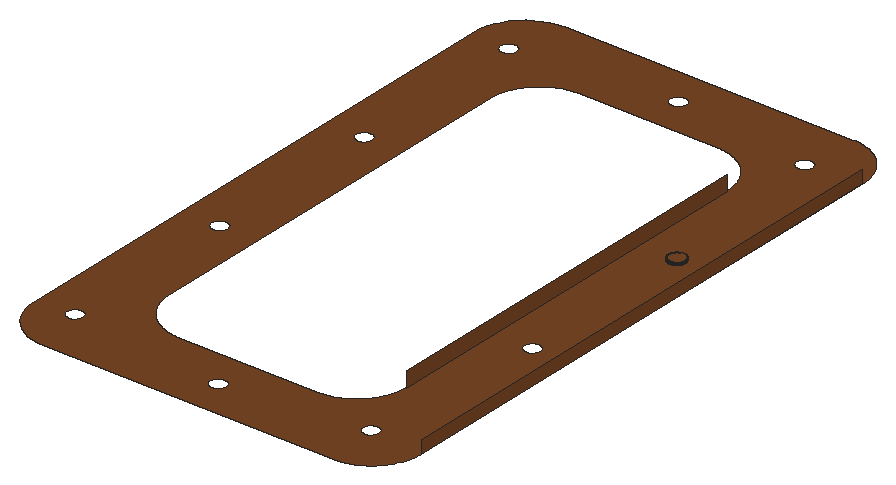
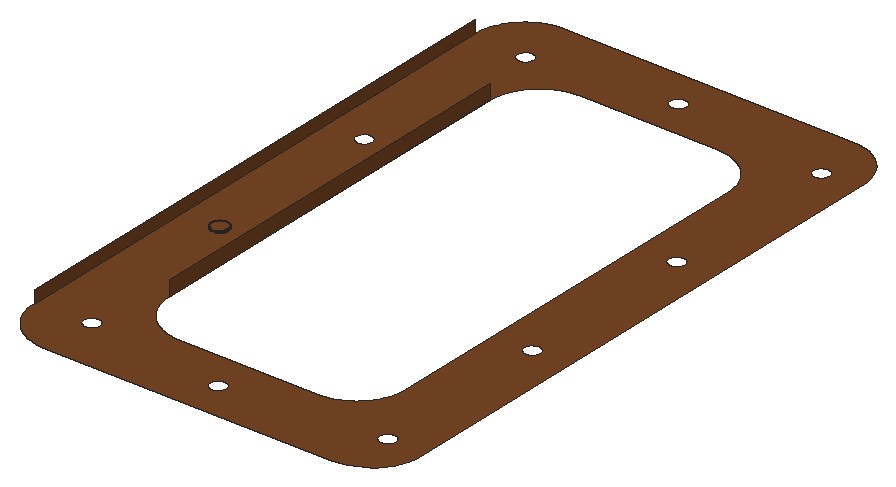
# SketchUp Ruby script. Lengths in inches.
U = 1.inch
M = Sketchup.active_model
def pt(a) = Geom::Point3d.new(a.map { |v| v * U })
def face(e, loops, mat)
  f = e.add_face(loops[0].map { |a| pt(a) })
  loops[1..].each { |l| e.add_face(l.map { |a| pt(a) }).erase! }
  f.material = f.back_material = mat if mat
  f
end
# faces: each face lists its corners as indices into pts; further lists are holes
def faces(e, pts, list, mat = nil) = list.each { |f| face(e, (f[0].is_a?(Array) ? f : [f]).map { |l| l.map { |i| pts[i] } }, mat) }
# xy, xz, yz: faces in a plane at the given z, y or x. An outline is a flat list of corners, or four numbers for a rectangle; further outlines are holes
def ring(l) = l.size == 4 ? [[l[0], l[1]], [l[2], l[1]], [l[2], l[3]], [l[0], l[3]]] : l.each_slice(2).to_a
def flat(e, list, mat, &to3) = list.each { |f| face(e, (f[0].is_a?(Array) ? f : [f]).map { |l| ring(l).map { |u, v| to3.(u, v) } }, mat) }
def xy(e, z, list, mat = nil) = flat(e, list, mat) { |x, y| [x, y, z] }
def xz(e, y, list, mat = nil) = flat(e, list, mat) { |x, z| [x, y, z] }
def yz(e, x, list, mat = nil) = flat(e, list, mat) { |y, z| [x, y, z] }
def lines(e, pts, list) = list.each { |a, b| e.add_line(pt(pts[a]), pt(pts[b])) }
# prism: a flat outline (further loops are holes) pulled along v
def prism(e, loops, v, mat = nil)
  f = face(e, loops, mat); d = Geom::Vector3d.new(v.map { |x| x * U })
  f.pushpull(f.normal.samedirection?(d) ? d.length : -d.length)
end
def box(e, o, s, mat = nil) = prism(e, [[o, [o[0] + s[0], o[1], o[2]], [o[0] + s[0], o[1] + s[1], o[2]], [o[0], o[1] + s[1], o[2]]]], [0, 0, s[2]], mat)
def at(x, y, z, deg = 0) = Geom::Transformation.translation(pt([x, y, z])) * Geom::Transformation.rotation(ORIGIN, Z_AXIS, deg.degrees)
def axes(o, x, y, z) = Geom::Transformation.new([*x, 0, *y, 0, *z, 0, *pt(o).to_a, 1])
def part(name) = M.definitions.add(name)
# library, detail: a bought-in or finely detailed component or shape, given as its bounding box
def library(name, o, s) = part(name).tap { |d| box(d.entities, o, s) }
def detail(e, o, s) = box(e.add_group.entities, o, s)
def put(e, d, t, mat = nil) = e.add_instance(d, t).tap { |i| i.material = mat if mat }
def group(e, t, mat = nil) = e.add_group.tap { |g| g.transformation = t; g.material = mat if mat }.entities
root = M.entities
M.materials.add("[Wood Veneer 01]3").color = [120, 70, 37]
xy(root,118,[[[75,27,73.43,27.1,71.89,27.41,70.41,27.91,69,28.61,67.69,29.48,66.51,30.51,65.48,31.69,64.61,33,63.91,34.41,63.41,35.89,63.1,37.43,63,39,63,171,63.1,172.57,63.41,174.11,63.91,175.59,64.61,177,65.48,178.31,66.51,179.49,67.69,180.52,69,181.39,70.41,182.09,71.89,182.59,73.43,182.9,75,183,144.3125,183,144.47,182.99,144.63,182.98,144.78,182.97,145.1,182.95,145.25,182.93,145.41,182.92,145.57,182.9,145.72,182.875,145.88,182.85,146.03,182.83,146.1875,182.8,146.34,182.77,146.49,182.74,146.65,182.7,146.8,182.67,146.95,182.63,147.11,182.59,147.41,182.51,147.86,182.36,148.01,182.3125,148.15,182.26,148.3,182.2,148.45,182.15,148.59,182.09,148.74,182.03,148.88,181.96,149.02,181.9,149.17,181.83,149.73,181.55,149.86,181.47,150,181.39,150.14,181.3125,150.27,181.23,150.4,181.15,150.54,181.0625,150.67,180.98,150.93,180.8,151.05,180.71,151.18,180.62,151.31,180.52,151.43,180.42,151.55,180.33,151.67,180.23,151.91,180.02,152.03,179.92,152.15,179.8125,152.26,179.7,152.375,179.6,152.49,179.49,152.6,179.375,152.7,179.26,152.8125,179.15,152.92,179.03,153.02,178.91,153.23,178.67,153.33,178.55,153.42,178.43,153.52,178.31,153.62,178.18,153.71,178.05,153.8,177.93,153.98,177.67,154.0625,177.54,154.15,177.4,154.23,177.27,154.3125,177.14,154.39,177,154.47,176.86,154.55,176.73,154.83,176.17,154.9,176.02,154.96,175.88,155.03,175.74,155.09,175.59,155.15,175.45,155.2,175.3,155.26,175.15,155.3125,175.01,155.36,174.86,155.51,174.41,155.59,174.11,155.63,173.95,155.67,173.8,155.7,173.65,155.74,173.49,155.77,173.34,155.8,173.1875,155.83,173.03,155.85,172.88,155.875,172.72,155.9,172.57,155.92,172.41,155.93,172.25,155.95,172.1,155.97,171.78,155.98,171.63,155.99,171.47,156,171.3125,156,38.6875,155.99,38.53,155.98,38.37,155.97,38.22,155.95,37.9,155.93,37.75,155.92,37.59,155.9,37.43,155.875,37.28,155.85,37.12,155.83,36.97,155.8,36.8125,155.77,36.66,155.74,36.51,155.7,36.35,155.67,36.2,155.63,36.05,155.59,35.89,155.51,35.59,155.36,35.14,155.3125,34.99,155.26,34.85,155.2,34.7,155.15,34.55,155.09,34.41,155.03,34.26,154.96,34.12,154.9,33.98,154.83,33.83,154.55,33.27,154.47,33.14,154.39,33,154.3125,32.86,154.23,32.73,154.15,32.6,154.0625,32.46,153.98,32.33,153.8,32.07,153.71,31.95,153.62,31.82,153.52,31.69,153.42,31.57,153.33,31.45,153.23,31.33,153.02,31.09,152.92,30.97,152.8125,30.85,152.7,30.74,152.6,30.625,152.49,30.51,152.375,30.4,152.26,30.3,152.15,30.1875,152.03,30.08,151.91,29.98,151.67,29.77,151.55,29.67,151.43,29.58,151.31,29.48,151.18,29.38,151.05,29.29,150.93,29.2,150.67,29.02,150.54,28.9375,150.4,28.85,150.27,28.77,150.14,28.6875,150,28.61,149.86,28.53,149.73,28.45,149.17,28.17,149.02,28.1,148.88,28.04,148.74,27.97,148.59,27.91,148.45,27.85,148.3,27.8,148.15,27.74,148.01,27.6875,147.86,27.64,147.41,27.49,147.11,27.41,146.95,27.37,146.8,27.33,146.65,27.3,146.49,27.26,146.34,27.23,146.1875,27.2,146.03,27.17,145.88,27.15,145.72,27.125,145.57,27.1,145.41,27.08,145.25,27.07,145.1,27.05,144.78,27.03,144.63,27.02,144.47,27.01,144.3125,27],[92.6875,45,126.3125,45,126.47,45.01,126.63,45.02,126.78,45.03,127.1,45.05,127.25,45.07,127.41,45.08,127.57,45.1,127.72,45.125,127.88,45.15,128.03,45.17,128.1875,45.2,128.34,45.23,128.49,45.26,128.65,45.3,128.8,45.33,128.95,45.37,129.11,45.41,129.41,45.49,129.86,45.64,130.01,45.6875,130.15,45.74,130.3,45.8,130.45,45.85,130.59,45.91,130.74,45.97,130.88,46.04,131.02,46.1,131.17,46.17,131.73,46.45,131.86,46.53,132,46.61,132.14,46.6875,132.27,46.77,132.4,46.85,132.54,46.9375,132.67,47.02,132.93,47.2,133.05,47.29,133.18,47.38,133.31,47.48,133.43,47.58,133.55,47.67,133.67,47.77,133.91,47.98,134.03,48.08,134.15,48.1875,134.26,48.3,134.375,48.4,134.49,48.51,134.6,48.625,134.7,48.74,134.8125,48.85,134.92,48.97,135.02,49.09,135.23,49.33,135.33,49.45,135.42,49.57,135.52,49.69,135.62,49.82,135.71,49.95,135.8,50.07,135.98,50.33,136.0625,50.46,136.15,50.6,136.23,50.73,136.3125,50.86,136.39,51,136.47,51.14,136.55,51.27,136.83,51.83,136.9,51.98,136.96,52.12,137.03,52.26,137.09,52.41,137.15,52.55,137.2,52.7,137.26,52.85,137.3125,52.99,137.36,53.14,137.51,53.59,137.59,53.89,137.63,54.05,137.67,54.2,137.7,54.35,137.74,54.51,137.77,54.66,137.8,54.8125,137.83,54.97,137.85,55.12,137.875,55.28,137.9,55.43,137.92,55.59,137.93,55.75,137.95,55.9,137.97,56.22,137.98,56.37,137.99,56.53,138,56.6875,138,153.3125,137.99,153.47,137.98,153.63,137.97,153.78,137.95,154.1,137.93,154.25,137.92,154.41,137.9,154.57,137.875,154.72,137.85,154.88,137.83,155.03,137.8,155.1875,137.77,155.34,137.74,155.49,137.7,155.65,137.67,155.8,137.63,155.95,137.59,156.11,137.51,156.41,137.36,156.86,137.3125,157.01,137.26,157.15,137.2,157.3,137.15,157.45,137.09,157.59,137.03,157.74,136.96,157.88,136.9,158.02,136.83,158.17,136.55,158.73,136.47,158.86,136.39,159,136.3125,159.14,136.23,159.27,136.15,159.4,136.0625,159.54,135.98,159.67,135.8,159.93,135.71,160.05,135.62,160.18,135.52,160.31,135.42,160.43,135.33,160.55,135.23,160.67,135.02,160.91,134.92,161.03,134.8125,161.15,134.7,161.26,134.6,161.375,134.49,161.49,134.375,161.6,134.26,161.7,134.15,161.8125,134.03,161.92,133.91,162.02,133.67,162.23,133.55,162.33,133.43,162.42,133.31,162.52,133.18,162.62,133.05,162.71,132.93,162.8,132.67,162.98,132.54,163.0625,132.4,163.15,132.27,163.23,132.14,163.3125,132,163.39,131.86,163.47,131.73,163.55,131.17,163.83,131.02,163.9,130.88,163.96,130.74,164.03,130.59,164.09,130.45,164.15,130.3,164.2,130.15,164.26,130.01,164.3125,129.86,164.36,129.41,164.51,129.11,164.59,128.95,164.63,128.8,164.67,128.65,164.7,128.49,164.74,128.34,164.77,128.1875,164.8,128.03,164.83,127.88,164.85,127.72,164.875,127.57,164.9,127.41,164.92,127.25,164.93,127.1,164.95,126.78,164.97,126.63,164.98,126.47,164.99,126.3125,165,92.6875,165,92.53,164.99,92.37,164.98,92.22,164.97,91.9,164.95,91.75,164.93,91.59,164.92,91.43,164.9,91.28,164.875,91.12,164.85,90.97,164.83,90.8125,164.8,90.66,164.77,90.51,164.74,90.35,164.7,90.2,164.67,90.05,164.63,89.89,164.59,89.59,164.51,89.14,164.36,88.99,164.3125,88.85,164.26,88.7,164.2,88.55,164.15,88.41,164.09,88.26,164.03,88.12,163.96,87.98,163.9,87.83,163.83,87.27,163.55,87.14,163.47,87,163.39,86.86,163.3125,86.73,163.23,86.6,163.15,86.46,163.0625,86.33,162.98,86.07,162.8,85.95,162.71,85.82,162.62,85.69,162.52,85.57,162.42,85.45,162.33,85.33,162.23,85.09,162.02,84.97,161.92,84.85,161.8125,84.74,161.7,84.625,161.6,84.51,161.49,84.4,161.375,84.3,161.26,84.1875,161.15,84.08,161.03,83.98,160.91,83.77,160.67,83.67,160.55,83.58,160.43,83.48,160.31,83.38,160.18,83.29,160.05,83.2,159.93,83.02,159.67,82.9375,159.54,82.85,159.4,82.77,159.27,82.6875,159.14,82.61,159,82.53,158.86,82.45,158.73,82.17,158.17,82.1,158.02,82.04,157.88,81.97,157.74,81.91,157.59,81.85,157.45,81.8,157.3,81.74,157.15,81.6875,157.01,81.64,156.86,81.49,156.41,81.41,156.11,81.37,155.95,81.33,155.8,81.3,155.65,81.26,155.49,81.23,155.34,81.2,155.1875,81.17,155.03,81.15,154.88,81.125,154.72,81.1,154.57,81.08,154.41,81.07,154.25,81.05,154.1,81.03,153.78,81.02,153.63,81.01,153.47,81,153.3125,81,56.6875,81.01,56.53,81.02,56.37,81.03,56.22,81.05,55.9,81.07,55.75,81.08,55.59,81.1,55.43,81.125,55.28,81.15,55.12,81.17,54.97,81.2,54.8125,81.23,54.66,81.26,54.51,81.3,54.35,81.33,54.2,81.37,54.05,81.41,53.89,81.49,53.59,81.64,53.14,81.6875,52.99,81.74,52.85,81.8,52.7,81.85,52.55,81.91,52.41,81.97,52.26,82.04,52.12,82.1,51.98,82.17,51.83,82.45,51.27,82.53,51.14,82.61,51,82.6875,50.86,82.77,50.73,82.85,50.6,82.9375,50.46,83.02,50.33,83.2,50.07,83.29,49.95,83.38,49.82,83.48,49.69,83.58,49.57,83.67,49.45,83.77,49.33,83.98,49.09,84.08,48.97,84.1875,48.85,84.3,48.74,84.4,48.625,84.51,48.51,84.625,48.4,84.74,48.3,84.85,48.1875,84.97,48.08,85.09,47.98,85.33,47.77,85.45,47.67,85.57,47.58,85.69,47.48,85.82,47.38,85.95,47.29,86.07,47.2,86.33,47.02,86.46,46.9375,86.6,46.85,86.73,46.77,86.86,46.6875,87,46.61,87.14,46.53,87.27,46.45,87.83,46.17,87.98,46.1,88.12,46.04,88.26,45.97,88.41,45.91,88.55,45.85,88.7,45.8,88.85,45.74,88.99,45.6875,89.14,45.64,89.59,45.49,89.89,45.41,90.05,45.37,90.2,45.33,90.35,45.3,90.51,45.26,90.66,45.23,90.8125,45.2,90.97,45.17,91.12,45.15,91.28,45.125,91.43,45.1,91.59,45.08,91.75,45.07,91.9,45.05,92.22,45.03,92.37,45.02,92.53,45.01],[71.99,81.33,72.07,81.33,72.15,81.34,72.24,81.35,72.32,81.36,72.48,81.39,72.56,81.41,72.8,81.5,72.875,81.54,72.95,81.57,73.02,81.62,73.1,81.66,73.16,81.71,73.3,81.81,73.36,81.87,73.42,81.92,73.48,81.98,73.53,82.05,73.58,82.11,73.73,82.32,73.77,82.39,73.8,82.47,73.84,82.55,73.9,82.7,73.96,82.94,73.98,83.03,74,83.19,74,83.44,73.99,83.53,73.97,83.69,73.95,83.78,73.93,83.86,73.91,83.9375,73.88,84.02,73.85,84.1,73.82,84.17,73.78,84.25,73.7,84.39,73.55,84.6,73.5,84.66,73.4375,84.72,73.38,84.78,73.32,84.84,73.25,84.89,73.1875,84.94,73.12,84.99,73.05,85.04,72.98,85.08,72.9,85.12,72.83,85.15,72.75,85.1875,72.67,85.22,72.59,85.24,72.51,85.27,72.43,85.29,72.35,85.3,72.26,85.32,72.18,85.33,71.85,85.33,71.76,85.32,71.68,85.31,71.36,85.23,71.2,85.17,71.05,85.09,70.98,85.05,70.9,85.01,70.84,84.96,70.7,84.86,70.52,84.68,70.47,84.62,70.42,84.55,70.37,84.49,70.27,84.35,70.23,84.27,70.2,84.2,70.16,84.12,70.1,83.96,70.02,83.64,70.01,83.56,70,83.47,70,83.22,70.02,83.06,70.03,82.97,70.09,82.73,70.18,82.49,70.26,82.35,70.3,82.27,70.35,82.2,70.4,82.14,70.45,82.07,70.5,82.01,70.5625,81.94,70.62,81.89,70.68,81.83,70.75,81.77,70.8125,81.72,70.88,81.68,70.95,81.63,71.02,81.59,71.1,81.55,71.17,81.51,71.41,81.42,71.65,81.36,71.74,81.35,71.82,81.34,71.9,81.34],[146.99,81.33,147.07,81.33,147.15,81.34,147.24,81.35,147.32,81.36,147.48,81.39,147.56,81.41,147.8,81.5,147.875,81.54,147.95,81.57,148.02,81.62,148.1,81.66,148.16,81.71,148.3,81.81,148.36,81.87,148.42,81.92,148.48,81.98,148.53,82.05,148.58,82.11,148.73,82.32,148.77,82.39,148.8,82.47,148.84,82.55,148.9,82.7,148.96,82.94,148.98,83.03,149,83.19,149,83.44,148.99,83.53,148.97,83.69,148.95,83.78,148.93,83.86,148.91,83.9375,148.88,84.02,148.85,84.1,148.82,84.17,148.78,84.25,148.7,84.39,148.55,84.6,148.5,84.66,148.4375,84.72,148.38,84.78,148.32,84.84,148.25,84.89,148.1875,84.94,148.12,84.99,148.05,85.04,147.98,85.08,147.9,85.12,147.83,85.15,147.75,85.1875,147.67,85.22,147.59,85.24,147.51,85.27,147.43,85.29,147.35,85.3,147.26,85.32,147.18,85.33,146.85,85.33,146.76,85.32,146.68,85.31,146.36,85.23,146.2,85.17,146.05,85.09,145.98,85.05,145.9,85.01,145.84,84.96,145.7,84.86,145.52,84.68,145.47,84.62,145.42,84.55,145.37,84.49,145.27,84.35,145.23,84.27,145.2,84.2,145.16,84.12,145.1,83.96,145.02,83.64,145.01,83.56,145,83.47,145,83.22,145.02,83.06,145.03,82.97,145.09,82.73,145.18,82.49,145.26,82.35,145.3,82.27,145.35,82.2,145.4,82.14,145.45,82.07,145.5,82.01,145.5625,81.94,145.62,81.89,145.68,81.83,145.75,81.77,145.8125,81.72,145.88,81.68,145.95,81.63,146.02,81.59,146.1,81.55,146.17,81.51,146.41,81.42,146.65,81.36,146.74,81.35,146.82,81.34,146.9,81.34],[142.9,168,143.07,168,143.15,168.01,143.24,168.01,143.32,168.03,143.4,168.04,143.56,168.08,143.8,168.17,143.875,168.2,143.95,168.24,144.02,168.28,144.1,168.33,144.16,168.375,144.23,168.42,144.3,168.48,144.36,168.53,144.48,168.65,144.53,168.71,144.73,168.99,144.77,169.0625,144.8,169.14,144.84,169.21,144.9,169.37,144.98,169.69,144.99,169.78,145,169.86,145,170.11,144.99,170.2,144.97,170.36,144.91,170.6,144.82,170.84,144.78,170.91,144.74,170.99,144.7,171.06,144.6,171.2,144.55,171.26,144.5,171.33,144.4375,171.39,144.38,171.45,144.32,171.5,144.25,171.56,144.1875,171.61,144.12,171.66,144.05,171.7,143.98,171.75,143.9,171.79,143.83,171.82,143.59,171.91,143.35,171.97,143.26,171.98,143.1,172,142.93,172,142.85,171.99,142.76,171.99,142.68,171.97,142.6,171.96,142.44,171.92,142.2,171.83,142.125,171.8,142.05,171.76,141.98,171.72,141.9,171.67,141.84,171.625,141.77,171.58,141.7,171.52,141.64,171.47,141.52,171.35,141.47,171.29,141.27,171.01,141.23,170.9375,141.2,170.86,141.16,170.79,141.1,170.63,141.02,170.31,141.01,170.22,141,170.14,141,169.89,141.01,169.8,141.03,169.64,141.09,169.4,141.18,169.16,141.22,169.09,141.26,169.01,141.3,168.94,141.4,168.8,141.45,168.74,141.5,168.67,141.5625,168.61,141.62,168.55,141.68,168.5,141.75,168.44,141.8125,168.39,141.88,168.34,141.95,168.3,142.02,168.25,142.1,168.21,142.17,168.18,142.41,168.09,142.65,168.03,142.74,168.02],[71.82,124.67,72.15,124.67,72.24,124.68,72.32,124.69,72.64,124.77,72.8,124.83,72.95,124.91,73.02,124.95,73.1,124.99,73.16,125.04,73.3,125.14,73.48,125.32,73.53,125.38,73.58,125.45,73.63,125.51,73.73,125.65,73.77,125.73,73.8,125.8,73.84,125.88,73.9,126.04,73.98,126.36,73.99,126.44,74,126.53,74,126.78,73.98,126.94,73.97,127.03,73.91,127.27,73.82,127.51,73.74,127.65,73.7,127.73,73.65,127.8,73.6,127.86,73.55,127.93,73.5,127.99,73.4375,128.06,73.38,128.11,73.32,128.17,73.25,128.23,73.1875,128.28,73.12,128.32,73.05,128.37,72.98,128.41,72.9,128.45,72.83,128.49,72.59,128.58,72.35,128.64,72.26,128.65,72.18,128.66,72.1,128.66,72.01,128.67,71.93,128.67,71.85,128.66,71.76,128.65,71.68,128.64,71.52,128.61,71.44,128.59,71.2,128.5,71.125,128.46,71.05,128.43,70.98,128.38,70.9,128.34,70.84,128.29,70.7,128.19,70.64,128.13,70.58,128.08,70.52,128.02,70.47,127.95,70.42,127.89,70.27,127.68,70.23,127.61,70.2,127.53,70.16,127.45,70.1,127.3,70.04,127.06,70.02,126.97,70,126.81,70,126.56,70.01,126.47,70.03,126.31,70.05,126.22,70.07,126.14,70.09,126.0625,70.12,125.98,70.15,125.9,70.18,125.83,70.22,125.75,70.3,125.61,70.45,125.4,70.5,125.34,70.5625,125.28,70.62,125.22,70.68,125.16,70.75,125.11,70.8125,125.06,70.88,125.01,70.95,124.96,71.02,124.92,71.1,124.88,71.17,124.85,71.25,124.8125,71.33,124.78,71.41,124.76,71.49,124.73,71.57,124.71,71.65,124.7,71.74,124.68],[71.9,168,72.07,168,72.15,168.01,72.24,168.01,72.32,168.03,72.4,168.04,72.56,168.08,72.8,168.17,72.875,168.2,72.95,168.24,73.02,168.28,73.1,168.33,73.16,168.375,73.23,168.42,73.3,168.48,73.36,168.53,73.48,168.65,73.53,168.71,73.73,168.99,73.77,169.0625,73.8,169.14,73.84,169.21,73.9,169.37,73.98,169.69,73.99,169.78,74,169.86,74,170.11,73.99,170.2,73.97,170.36,73.91,170.6,73.82,170.84,73.78,170.91,73.74,170.99,73.7,171.06,73.6,171.2,73.55,171.26,73.5,171.33,73.4375,171.39,73.38,171.45,73.32,171.5,73.25,171.56,73.1875,171.61,73.12,171.66,73.05,171.7,72.98,171.75,72.9,171.79,72.83,171.82,72.59,171.91,72.35,171.97,72.26,171.98,72.1,172,71.93,172,71.85,171.99,71.76,171.99,71.68,171.97,71.6,171.96,71.44,171.92,71.2,171.83,71.125,171.8,71.05,171.76,70.98,171.72,70.9,171.67,70.84,171.625,70.77,171.58,70.7,171.52,70.64,171.47,70.52,171.35,70.47,171.29,70.27,171.01,70.23,170.9375,70.2,170.86,70.16,170.79,70.1,170.63,70.02,170.31,70.01,170.22,70,170.14,70,169.89,70.01,169.8,70.03,169.64,70.09,169.4,70.18,169.16,70.22,169.09,70.26,169.01,70.3,168.94,70.4,168.8,70.45,168.74,70.5,168.67,70.5625,168.61,70.62,168.55,70.68,168.5,70.75,168.44,70.8125,168.39,70.88,168.34,70.95,168.3,71.02,168.25,71.1,168.21,71.17,168.18,71.41,168.09,71.65,168.03,71.74,168.02],[146.82,124.67,147.15,124.67,147.24,124.68,147.32,124.69,147.64,124.77,147.8,124.83,147.95,124.91,148.02,124.95,148.1,124.99,148.16,125.04,148.3,125.14,148.48,125.32,148.53,125.38,148.58,125.45,148.63,125.51,148.73,125.65,148.77,125.73,148.8,125.8,148.84,125.88,148.9,126.04,148.98,126.36,148.99,126.44,149,126.53,149,126.78,148.98,126.94,148.97,127.03,148.91,127.27,148.82,127.51,148.74,127.65,148.7,127.73,148.65,127.8,148.6,127.86,148.55,127.93,148.5,127.99,148.4375,128.06,148.38,128.11,148.32,128.17,148.25,128.23,148.1875,128.28,148.12,128.32,148.05,128.37,147.98,128.41,147.9,128.45,147.83,128.49,147.59,128.58,147.35,128.64,147.26,128.65,147.18,128.66,147.1,128.66,147.01,128.67,146.93,128.67,146.85,128.66,146.76,128.65,146.68,128.64,146.52,128.61,146.44,128.59,146.2,128.5,146.125,128.46,146.05,128.43,145.98,128.38,145.9,128.34,145.84,128.29,145.7,128.19,145.64,128.13,145.58,128.08,145.52,128.02,145.47,127.95,145.42,127.89,145.27,127.68,145.23,127.61,145.2,127.53,145.16,127.45,145.1,127.3,145.04,127.06,145.02,126.97,145,126.81,145,126.56,145.01,126.47,145.03,126.31,145.05,126.22,145.07,126.14,145.09,126.0625,145.12,125.98,145.15,125.9,145.18,125.83,145.22,125.75,145.3,125.61,145.45,125.4,145.5,125.34,145.5625,125.28,145.62,125.22,145.68,125.16,145.75,125.11,145.8125,125.06,145.88,125.01,145.95,124.96,146.02,124.92,146.1,124.88,146.17,124.85,146.25,124.8125,146.33,124.78,146.41,124.76,146.49,124.73,146.57,124.71,146.65,124.7,146.74,124.68],[109.4,34,109.57,34,109.65,34.01,109.74,34.01,109.82,34.03,109.9,34.04,110.06,34.08,110.3,34.17,110.375,34.2,110.45,34.24,110.52,34.28,110.6,34.33,110.66,34.375,110.73,34.42,110.8,34.48,110.86,34.53,110.98,34.65,111.03,34.71,111.23,34.99,111.27,35.0625,111.3,35.14,111.34,35.21,111.4,35.37,111.48,35.69,111.49,35.78,111.5,35.86,111.5,36.11,111.49,36.2,111.47,36.36,111.41,36.6,111.32,36.84,111.28,36.91,111.24,36.99,111.2,37.06,111.1,37.2,111.05,37.26,111,37.33,110.9375,37.39,110.88,37.45,110.82,37.5,110.75,37.56,110.6875,37.61,110.62,37.66,110.55,37.7,110.48,37.75,110.4,37.79,110.33,37.82,110.09,37.91,109.85,37.97,109.76,37.98,109.6,38,109.43,38,109.35,37.99,109.26,37.99,109.18,37.97,109.1,37.96,108.94,37.92,108.7,37.83,108.625,37.8,108.55,37.76,108.48,37.72,108.4,37.67,108.34,37.625,108.27,37.58,108.2,37.52,108.14,37.47,108.02,37.35,107.97,37.29,107.77,37.01,107.73,36.9375,107.7,36.86,107.66,36.79,107.6,36.63,107.52,36.31,107.51,36.22,107.5,36.14,107.5,35.89,107.51,35.8,107.53,35.64,107.59,35.4,107.68,35.16,107.72,35.09,107.76,35.01,107.8,34.94,107.9,34.8,107.95,34.74,108,34.67,108.0625,34.61,108.12,34.55,108.18,34.5,108.25,34.44,108.3125,34.39,108.38,34.34,108.45,34.3,108.52,34.25,108.6,34.21,108.67,34.18,108.91,34.09,109.15,34.03,109.24,34.02],[142.9,38,143.07,38,143.15,38.01,143.24,38.01,143.32,38.03,143.4,38.04,143.56,38.08,143.8,38.17,143.875,38.2,143.95,38.24,144.02,38.28,144.1,38.33,144.16,38.375,144.23,38.42,144.3,38.48,144.36,38.53,144.48,38.65,144.53,38.71,144.73,38.99,144.77,39.0625,144.8,39.14,144.84,39.21,144.9,39.37,144.98,39.69,144.99,39.78,145,39.86,145,40.11,144.99,40.2,144.97,40.36,144.91,40.6,144.82,40.84,144.78,40.91,144.74,40.99,144.7,41.06,144.6,41.2,144.55,41.26,144.5,41.33,144.4375,41.39,144.38,41.45,144.32,41.5,144.25,41.56,144.1875,41.61,144.12,41.66,144.05,41.7,143.98,41.75,143.9,41.79,143.83,41.82,143.59,41.91,143.35,41.97,143.26,41.98,143.1,42,142.93,42,142.85,41.99,142.76,41.99,142.68,41.97,142.6,41.96,142.44,41.92,142.2,41.83,142.125,41.8,142.05,41.76,141.98,41.72,141.9,41.67,141.84,41.625,141.77,41.58,141.7,41.52,141.64,41.47,141.52,41.35,141.47,41.29,141.27,41.01,141.23,40.9375,141.2,40.86,141.16,40.79,141.1,40.63,141.02,40.31,141.01,40.22,141,40.14,141,39.89,141.01,39.8,141.03,39.64,141.09,39.4,141.18,39.16,141.22,39.09,141.26,39.01,141.3,38.94,141.4,38.8,141.45,38.74,141.5,38.67,141.5625,38.61,141.62,38.55,141.68,38.5,141.75,38.44,141.8125,38.39,141.88,38.34,141.95,38.3,142.02,38.25,142.1,38.21,142.17,38.18,142.41,38.09,142.65,38.03,142.74,38.02],[109.4,172,109.57,172,109.65,172.01,109.74,172.01,109.82,172.03,109.9,172.04,110.06,172.08,110.3,172.17,110.375,172.2,110.45,172.24,110.52,172.28,110.6,172.33,110.66,172.375,110.73,172.42,110.8,172.48,110.86,172.53,110.98,172.65,111.03,172.71,111.23,172.99,111.27,173.0625,111.3,173.14,111.34,173.21,111.4,173.37,111.48,173.69,111.49,173.78,111.5,173.86,111.5,174.11,111.49,174.2,111.47,174.36,111.41,174.6,111.32,174.84,111.28,174.91,111.24,174.99,111.2,175.06,111.1,175.2,111.05,175.26,111,175.33,110.9375,175.39,110.88,175.45,110.82,175.5,110.75,175.56,110.6875,175.61,110.62,175.66,110.55,175.7,110.48,175.75,110.4,175.79,110.33,175.82,110.09,175.91,109.85,175.97,109.76,175.98,109.6,176,109.43,176,109.35,175.99,109.26,175.99,109.18,175.97,109.1,175.96,108.94,175.92,108.7,175.83,108.625,175.8,108.55,175.76,108.48,175.72,108.4,175.67,108.34,175.625,108.27,175.58,108.2,175.52,108.14,175.47,108.02,175.35,107.97,175.29,107.77,175.01,107.73,174.9375,107.7,174.86,107.66,174.79,107.6,174.63,107.52,174.31,107.51,174.22,107.5,174.14,107.5,173.89,107.51,173.8,107.53,173.64,107.59,173.4,107.68,173.16,107.72,173.09,107.76,173.01,107.8,172.94,107.9,172.8,107.95,172.74,108,172.67,108.0625,172.61,108.12,172.55,108.18,172.5,108.25,172.44,108.3125,172.39,108.38,172.34,108.45,172.3,108.52,172.25,108.6,172.21,108.67,172.18,108.91,172.09,109.15,172.03,109.24,172.02],[71.9,38,72.07,38,72.15,38.01,72.24,38.01,72.32,38.03,72.4,38.04,72.56,38.08,72.8,38.17,72.875,38.2,72.95,38.24,73.02,38.28,73.1,38.33,73.16,38.375,73.23,38.42,73.3,38.48,73.36,38.53,73.48,38.65,73.53,38.71,73.73,38.99,73.77,39.0625,73.8,39.14,73.84,39.21,73.9,39.37,73.98,39.69,73.99,39.78,74,39.86,74,40.11,73.99,40.2,73.97,40.36,73.91,40.6,73.82,40.84,73.78,40.91,73.74,40.99,73.7,41.06,73.6,41.2,73.55,41.26,73.5,41.33,73.4375,41.39,73.38,41.45,73.32,41.5,73.25,41.56,73.1875,41.61,73.12,41.66,73.05,41.7,72.98,41.75,72.9,41.79,72.83,41.82,72.59,41.91,72.35,41.97,72.26,41.98,72.1,42,71.93,42,71.85,41.99,71.76,41.99,71.68,41.97,71.6,41.96,71.44,41.92,71.2,41.83,71.125,41.8,71.05,41.76,70.98,41.72,70.9,41.67,70.84,41.625,70.77,41.58,70.7,41.52,70.64,41.47,70.52,41.35,70.47,41.29,70.27,41.01,70.23,40.9375,70.2,40.86,70.16,40.79,70.1,40.63,70.02,40.31,70.01,40.22,70,40.14,70,39.89,70.01,39.8,70.03,39.64,70.09,39.4,70.18,39.16,70.22,39.09,70.26,39.01,70.3,38.94,70.4,38.8,70.45,38.74,70.5,38.67,70.5625,38.61,70.62,38.55,70.68,38.5,70.75,38.44,70.8125,38.39,70.88,38.34,70.95,38.3,71.02,38.25,71.1,38.21,71.17,38.18,71.41,38.09,71.65,38.03,71.74,38.02]]],"[Wood Veneer 01]3")
xy(root,118.5,[[146.82,124.67,146.74,124.68,146.65,124.7,146.57,124.71,146.49,124.73,146.41,124.76,146.33,124.78,146.25,124.8125,146.17,124.85,146.1,124.88,146.02,124.92,145.95,124.96,145.88,125.01,145.8125,125.06,145.75,125.11,145.68,125.16,145.62,125.22,145.5625,125.28,145.5,125.34,145.45,125.4,145.3,125.61,145.22,125.75,145.18,125.83,145.15,125.9,145.12,125.98,145.09,126.0625,145.07,126.14,145.05,126.22,145.03,126.31,145.01,126.47,145,126.56,145,126.81,145.02,126.97,145.04,127.06,145.1,127.3,145.16,127.45,145.2,127.53,145.23,127.61,145.27,127.68,145.42,127.89,145.47,127.95,145.52,128.02,145.58,128.08,145.64,128.13,145.7,128.19,145.84,128.29,145.9,128.34,145.98,128.38,146.05,128.43,146.125,128.46,146.2,128.5,146.44,128.59,146.52,128.61,146.68,128.64,146.76,128.65,146.85,128.66,146.93,128.67,147.01,128.67,147.1,128.66,147.18,128.66,147.26,128.65,147.35,128.64,147.59,128.58,147.83,128.49,147.9,128.45,147.98,128.41,148.05,128.37,148.12,128.32,148.1875,128.28,148.25,128.23,148.32,128.17,148.38,128.11,148.4375,128.06,148.5,127.99,148.55,127.93,148.6,127.86,148.65,127.8,148.7,127.73,148.74,127.65,148.82,127.51,148.91,127.27,148.97,127.03,148.98,126.94,149,126.78,149,126.53,148.99,126.44,148.98,126.36,148.9,126.04,148.84,125.88,148.8,125.8,148.77,125.73,148.73,125.65,148.63,125.51,148.58,125.45,148.53,125.38,148.48,125.32,148.3,125.14,148.16,125.04,148.1,124.99,148.02,124.95,147.95,124.91,147.8,124.83,147.64,124.77,147.32,124.69,147.24,124.68,147.15,124.67]],"[Wood Veneer 01]3")
xz(root,124.67,[[146.82,118,146.9,118.5],[146.9,118,146.99,118.5],[146.99,118,147.07,118.5],[147.07,118,147.15,118.5]],"[Wood Veneer 01]3")
yz(root,138,[[57,118,153,121.5]],"[Wood Veneer 01]3")
yz(root,145,[[126.56,118,126.64,118.5],[126.64,118,126.72,118.5],[126.72,118,126.81,118.5]],"[Wood Veneer 01]3")
yz(root,149,[[126.53,118,126.61,118.5],[126.61,118,126.69,118.5],[126.69,118,126.78,118.5]],"[Wood Veneer 01]3")
yz(root,156,[[39,118,171,121]],"[Wood Veneer 01]3")
p = [[146.49,124.73,118],[146.41,124.76,118],[146.41,124.76,118.5],[146.49,124.73,118.5],[146.57,124.71,118],[146.57,124.71,118.5],
  [146.65,124.7,118],[146.65,124.7,118.5],[146.82,124.67,118],[146.74,124.68,118],[146.74,124.68,118.5],[146.82,124.67,118.5],
  [147.24,124.68,118],[147.15,124.67,118],[147.15,124.67,118.5],[147.24,124.68,118.5],[147.32,124.69,118],[147.32,124.69,118.5],
  [147.4,124.71,118],[147.4,124.71,118.5],[147.48,124.73,118],[147.48,124.73,118.5],[147.56,124.75,118],[147.56,124.75,118.5],
  [147.64,124.77,118],[147.64,124.77,118.5],[146.17,124.85,118],[146.1,124.88,118],[146.1,124.88,118.5],[146.17,124.85,118.5],
  [146.25,124.8125,118],[146.25,124.8125,118.5],[146.33,124.78,118],[146.33,124.78,118.5],[147.72,124.8,118],[147.72,124.8,118.5],
  [147.8,124.83,118],[147.8,124.83,118.5],[147.875,124.87,118],[147.875,124.87,118.5],[146.02,124.92,118],[146.02,124.92,118.5],
  [145.95,124.96,118],[145.95,124.96,118.5],[147.95,124.91,118],[147.95,124.91,118.5],[148.02,124.95,118],[148.02,124.95,118.5],
  [148.1,124.99,118],[148.1,124.99,118.5],[145.88,125.01,118],[145.8125,125.06,118],[145.8125,125.06,118.5],[145.88,125.01,118.5],
  [148.16,125.04,118],[148.16,125.04,118.5],[148.23,125.09,118],[148.23,125.09,118.5],[145.75,125.11,118],[145.75,125.11,118.5],
  [145.68,125.16,118],[145.68,125.16,118.5],[148.3,125.14,118],[148.3,125.14,118.5],[148.36,125.2,118],[148.36,125.2,118.5],
  [145.62,125.22,118],[145.62,125.22,118.5],[145.5625,125.28,118],[145.5625,125.28,118.5],[148.42,125.26,118],[148.42,125.26,118.5],
  [145.5,125.34,118],[145.5,125.34,118.5],[145.45,125.4,118],[145.45,125.4,118.5],[148.48,125.32,118],[148.48,125.32,118.5],
  [148.53,125.38,118],[148.53,125.38,118.5],[145.4,125.47,118],[145.4,125.47,118.5],[148.58,125.45,118],[148.58,125.45,118.5],
  [148.63,125.51,118],[148.63,125.51,118.5],[145.35,125.54,118],[145.35,125.54,118.5],[145.3,125.61,118],[145.3,125.61,118.5],
  [148.68,125.58,118],[148.68,125.58,118.5],[145.26,125.68,118],[145.26,125.68,118.5],[148.73,125.65,118],[148.73,125.65,118.5],
  [145.22,125.75,118],[145.22,125.75,118.5],[148.77,125.73,118],[148.77,125.73,118.5],[148.8,125.8,118],[148.8,125.8,118.5],
  [145.18,125.83,118],[145.18,125.83,118.5],[145.15,125.9,118],[145.15,125.9,118.5],[148.84,125.88,118],[148.84,125.88,118.5],
  [145.12,125.98,118],[145.12,125.98,118.5],[148.87,125.96,118],[148.87,125.96,118.5],[145.09,126.0625,118],[145.09,126.0625,118.5],
  [148.9,126.04,118],[148.9,126.04,118.5],[148.92,126.12,118],[148.92,126.12,118.5],[145.07,126.14,118],[145.05,126.22,118],
  [145.05,126.22,118.5],[145.07,126.14,118.5],[148.94,126.2,118],[148.94,126.2,118.5],[145.03,126.31,118],[145.03,126.31,118.5],
  [148.96,126.28,118],[148.96,126.28,118.5],[145.02,126.39,118],[145.02,126.39,118.5],[148.98,126.36,118],[148.98,126.36,118.5],
  [145.01,126.47,118],[145.01,126.47,118.5],[148.99,126.44,118],[148.99,126.44,118.5],[149,126.53,118],[149,126.53,118.5],
  [145,126.56,118],[145,126.56,118.5],[145,126.81,118],[145.01,126.89,118],[145.01,126.89,118.5],[145,126.81,118.5],
  [148.99,126.86,118],[149,126.78,118],[149,126.78,118.5],[148.99,126.86,118.5],[145.02,126.97,118],[145.02,126.97,118.5],
  [148.98,126.94,118],[148.98,126.94,118.5],[148.97,127.03,118],[148.97,127.03,118.5],[145.04,127.06,118],[145.04,127.06,118.5],
  [148.95,127.11,118],[148.95,127.11,118.5],[145.06,127.14,118],[145.06,127.14,118.5],[145.08,127.22,118],[145.08,127.22,118.5],
  [148.93,127.19,118],[148.93,127.19,118.5],[145.1,127.3,118],[145.1,127.3,118.5],[148.91,127.27,118],[148.91,127.27,118.5],
  [145.13,127.375,118],[145.13,127.375,118.5],[148.88,127.35,118],[148.88,127.35,118.5],[145.16,127.45,118],[145.16,127.45,118.5],
  [148.85,127.43,118],[148.85,127.43,118.5],[148.82,127.51,118],[148.82,127.51,118.5],[145.2,127.53,118],[145.2,127.53,118.5],
  [145.23,127.61,118],[145.23,127.61,118.5],[148.78,127.58,118],[148.78,127.58,118.5],[145.27,127.68,118],[145.27,127.68,118.5],
  [148.74,127.65,118],[148.74,127.65,118.5],[145.32,127.75,118],[145.32,127.75,118.5],[148.7,127.73,118],[148.7,127.73,118.5],
  [148.65,127.8,118],[148.65,127.8,118.5],[145.37,127.82,118],[145.37,127.82,118.5],[145.42,127.89,118],[145.42,127.89,118.5],
  [148.6,127.86,118],[148.6,127.86,118.5],[145.47,127.95,118],[145.47,127.95,118.5],[148.55,127.93,118],[148.55,127.93,118.5],
  [148.5,127.99,118],[148.5,127.99,118.5],[145.52,128.02,118],[145.52,128.02,118.5],[145.58,128.08,118],[145.58,128.08,118.5],
  [148.4375,128.06,118],[148.4375,128.06,118.5],[145.64,128.13,118],[145.64,128.13,118.5],[145.7,128.19,118],[145.7,128.19,118.5],
  [148.32,128.17,118],[148.38,128.11,118],[148.38,128.11,118.5],[148.32,128.17,118.5],[145.77,128.24,118],[145.77,128.24,118.5],
  [145.84,128.29,118],[145.84,128.29,118.5],[148.1875,128.28,118],[148.25,128.23,118],[148.25,128.23,118.5],[148.1875,128.28,118.5],
  [145.9,128.34,118],[145.9,128.34,118.5],[145.98,128.38,118],[145.98,128.38,118.5],[148.05,128.37,118],[148.12,128.32,118],
  [148.12,128.32,118.5],[148.05,128.37,118.5],[146.05,128.43,118],[146.05,128.43,118.5],[146.125,128.46,118],[146.125,128.46,118.5],
  [147.9,128.45,118],[147.98,128.41,118],[147.98,128.41,118.5],[147.9,128.45,118.5],[146.2,128.5,118],[146.2,128.5,118.5],
  [146.28,128.53,118],[146.28,128.53,118.5],[146.36,128.56,118],[146.36,128.56,118.5],[147.75,128.52,118],[147.83,128.49,118],
  [147.83,128.49,118.5],[147.75,128.52,118.5],[147.67,128.55,118],[147.67,128.55,118.5],[146.44,128.59,118],[146.44,128.59,118.5],
  [147.51,128.6,118],[147.59,128.58,118],[147.59,128.58,118.5],[147.51,128.6,118.5]]
faces(root,p,[[0,1,2,3],[4,0,3,5],[6,4,5,7],[8,9,10,11],[9,6,7,10],[12,13,14,15],[16,12,15,17],[18,16,17,19],
  [20,18,19,21],[22,20,21,23],[24,22,23,25],[26,27,28,29],[30,26,29,31],[1,32,33,2],[32,30,31,33],[34,24,25,35],
  [36,34,35,37],[38,36,37,39],[27,40,41,28],[40,42,43,41],[44,38,39,45],[46,44,45,47],[48,46,47,49],[50,51,52,53],
  [42,50,53,43],[54,48,49,55],[56,54,55,57],[51,58,59,52],[58,60,61,59],[62,56,57,63],[64,62,63,65],[60,66,67,61],
  [66,68,69,67],[70,64,65,71],[68,72,73,69],[72,74,75,73],[76,70,71,77],[78,76,77,79],[74,80,81,75],[82,78,79,83],
  [84,82,83,85],[80,86,87,81],[86,88,89,87],[90,84,85,91],[88,92,93,89],[94,90,91,95],[92,96,97,93],[98,94,95,99],
  [100,98,99,101],[96,102,103,97],[102,104,105,103],[106,100,101,107],[104,108,109,105],[110,106,107,111],[108,112,113,109],[114,110,111,115],
  [116,114,115,117],[118,119,120,121],[112,118,121,113],[122,116,117,123],[119,124,125,120],[126,122,123,127],[124,128,129,125],[130,126,127,131],
  [128,132,133,129],[134,130,131,135],[136,134,135,137],[132,138,139,133],[140,141,142,143],[144,145,146,147],[141,148,149,142],[150,144,147,151],
  [152,150,151,153],[148,154,155,149],[156,152,153,157],[154,158,159,155],[158,160,161,159],[162,156,157,163],[160,164,165,161],[166,162,163,167],
  [164,168,169,165],[170,166,167,171],[168,172,173,169],[174,170,171,175],[176,174,175,177],[172,178,179,173],[178,180,181,179],[182,176,177,183],
  [180,184,185,181],[186,182,183,187],[184,188,189,185],[190,186,187,191],[192,190,191,193],[188,194,195,189],[194,196,197,195],[198,192,193,199],
  [196,200,201,197],[202,198,199,203],[204,202,203,205],[200,206,207,201],[206,208,209,207],[210,204,205,211],[208,212,213,209],[212,214,215,213],
  [216,217,218,219],[217,210,211,218],[214,220,221,215],[220,222,223,221],[224,225,226,227],[225,216,219,226],[222,228,229,223],[228,230,231,229],
  [232,233,234,235],[233,224,227,234],[230,236,237,231],[236,238,239,237],[240,241,242,243],[241,232,235,242],[238,244,245,239],[244,246,247,245],
  [246,248,249,247],[250,251,252,253],[254,250,253,255],[251,240,243,252],[248,256,257,249],[258,259,260,261],[259,254,255,260]],"[Wood Veneer 01]3")
